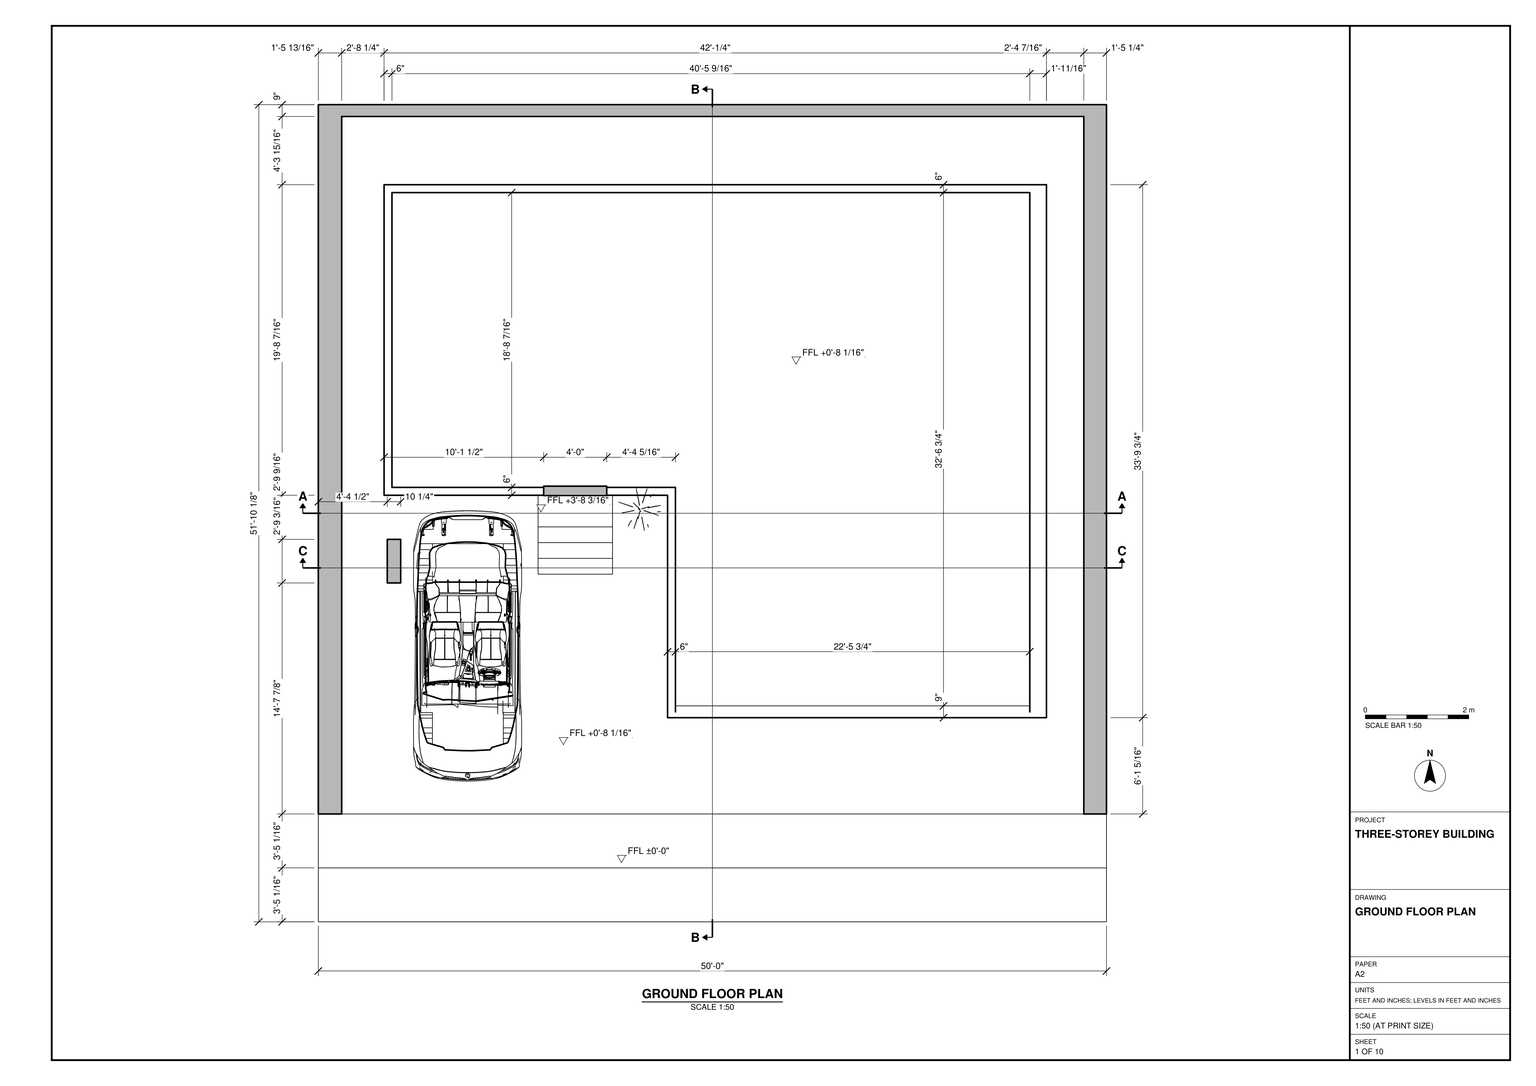
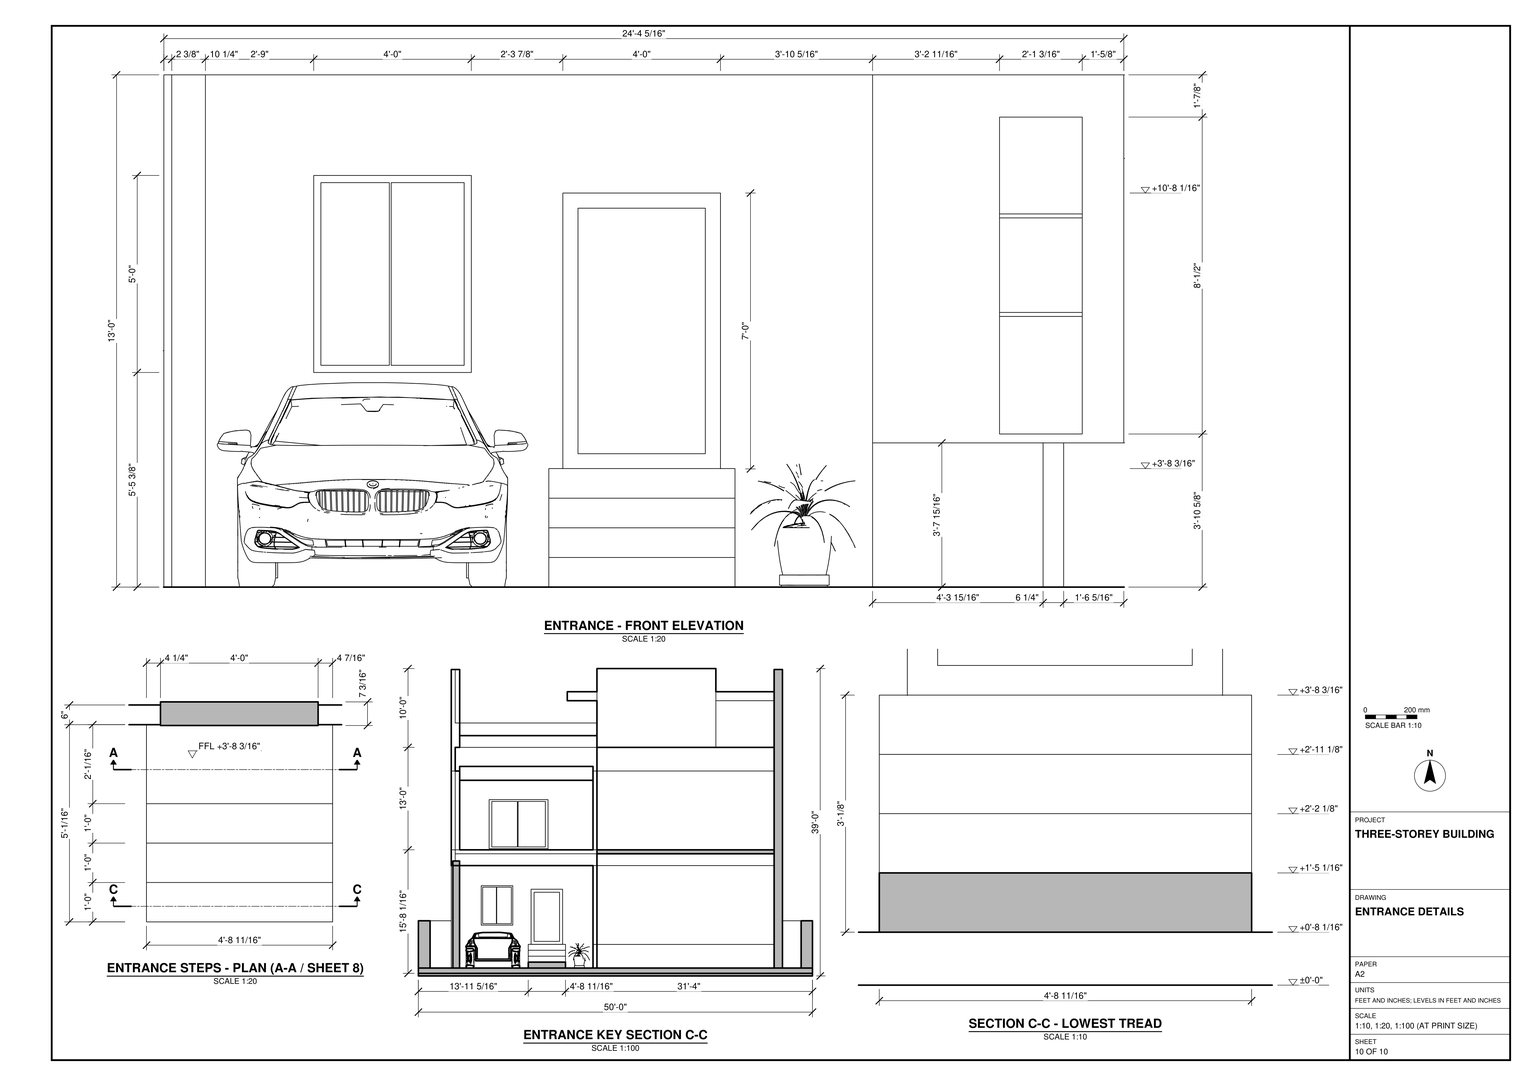
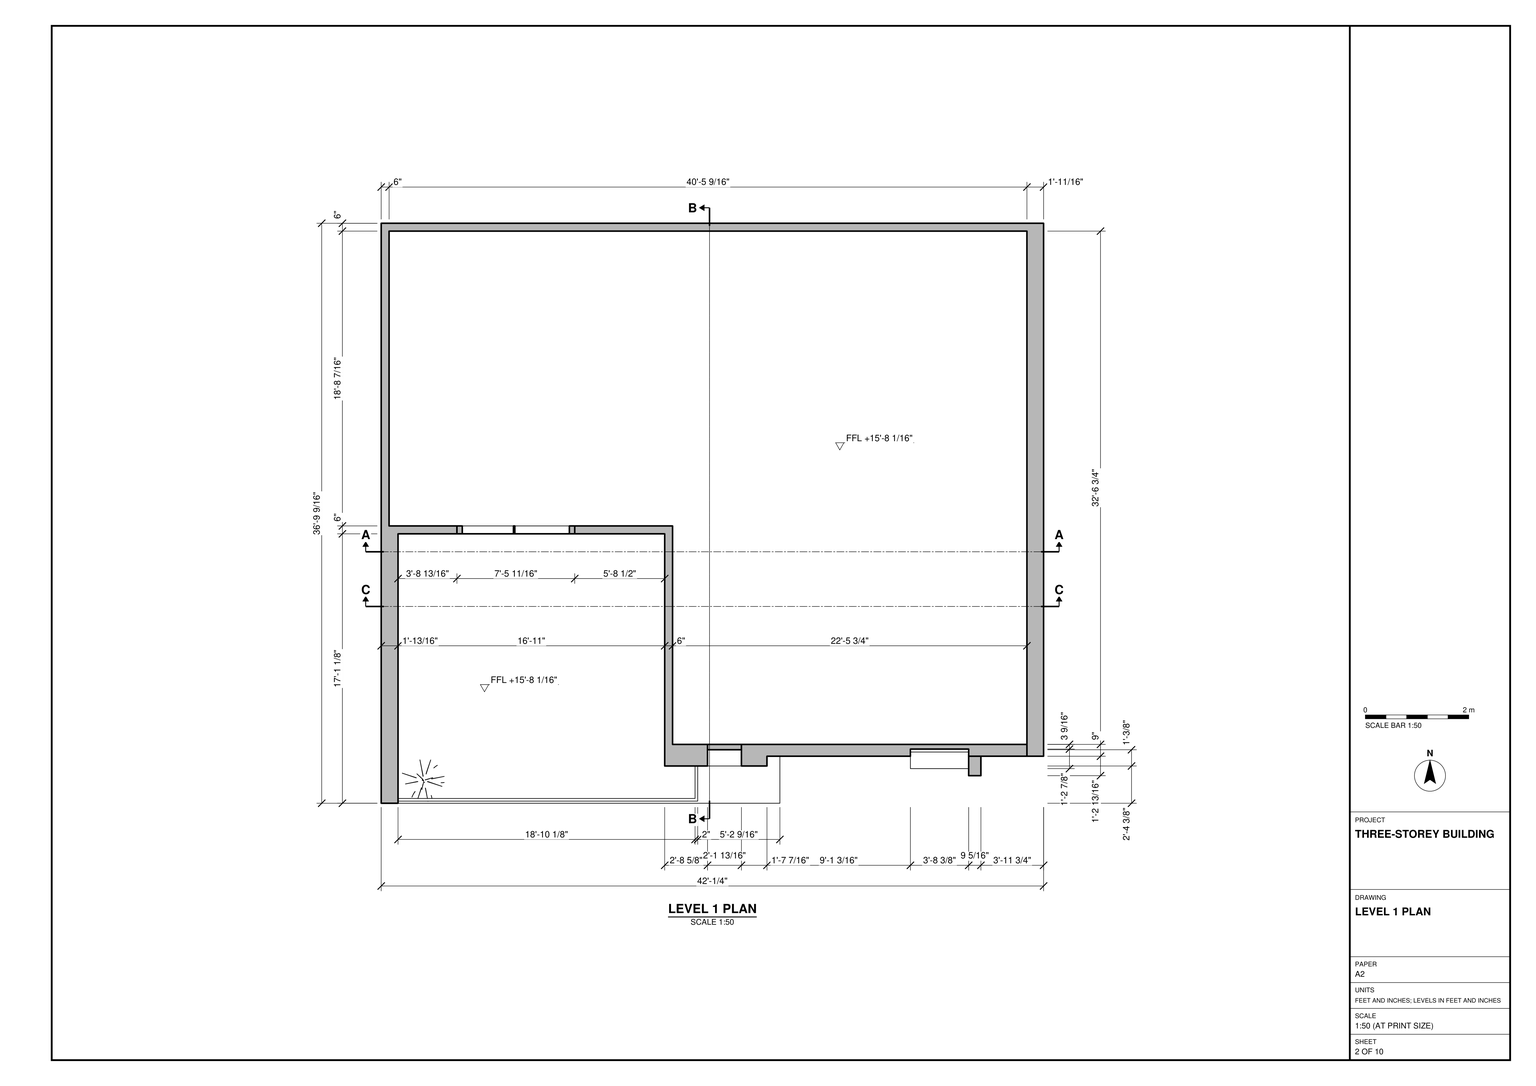
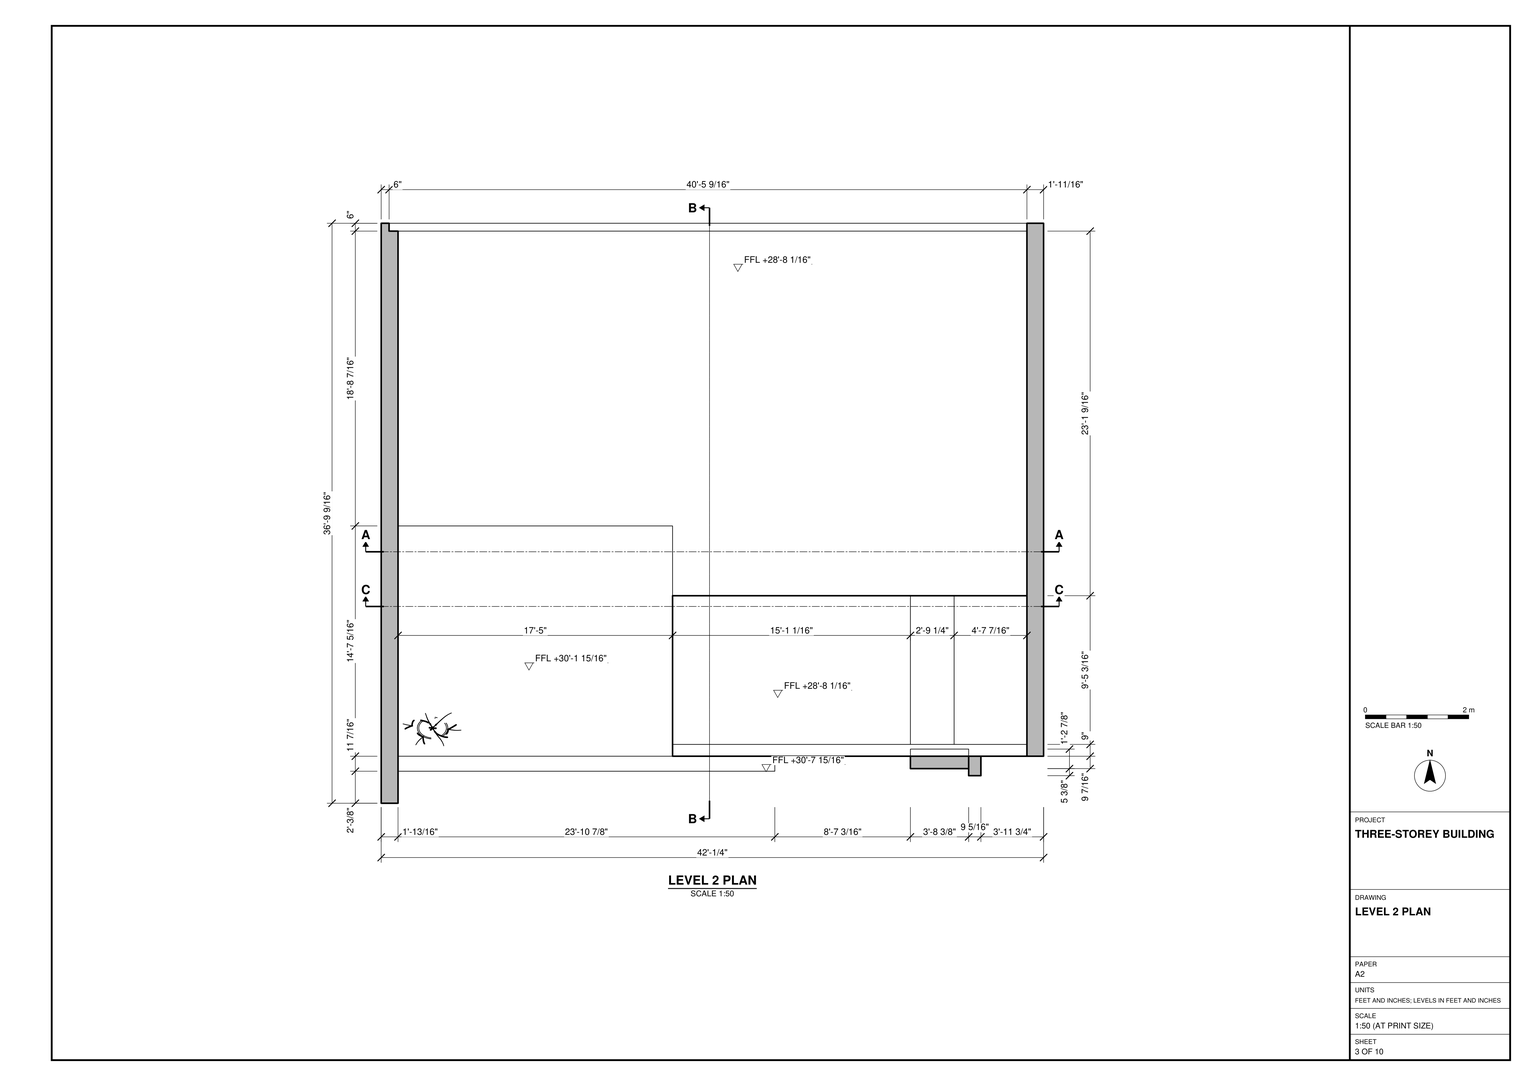
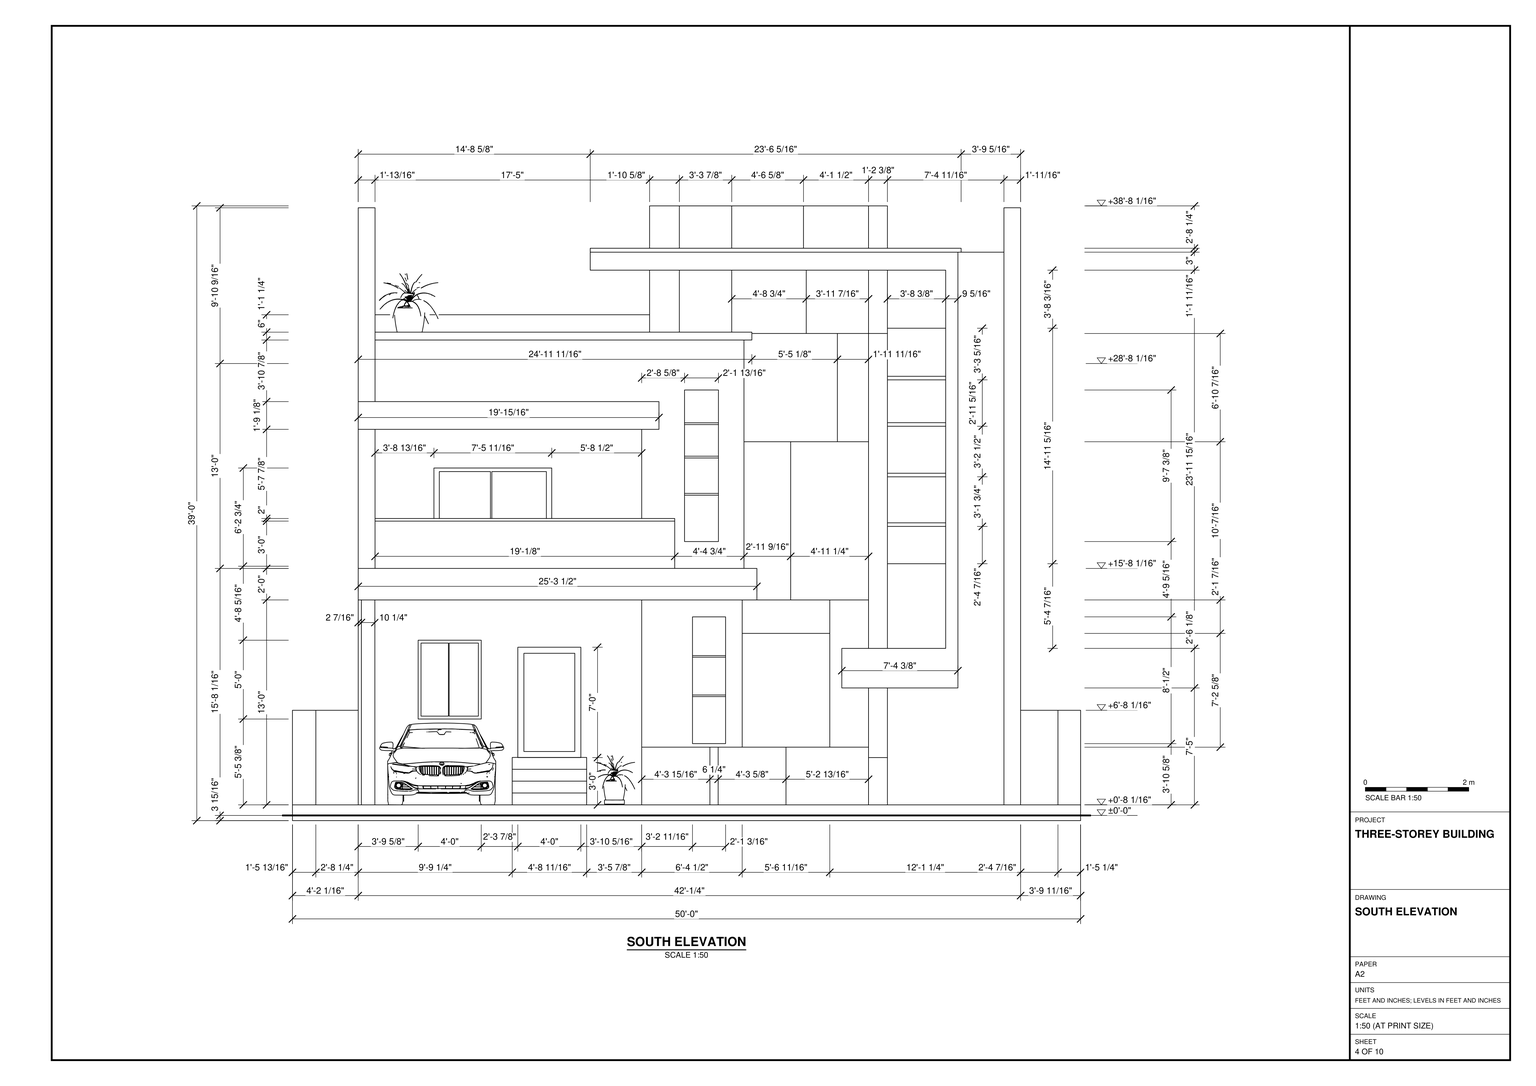
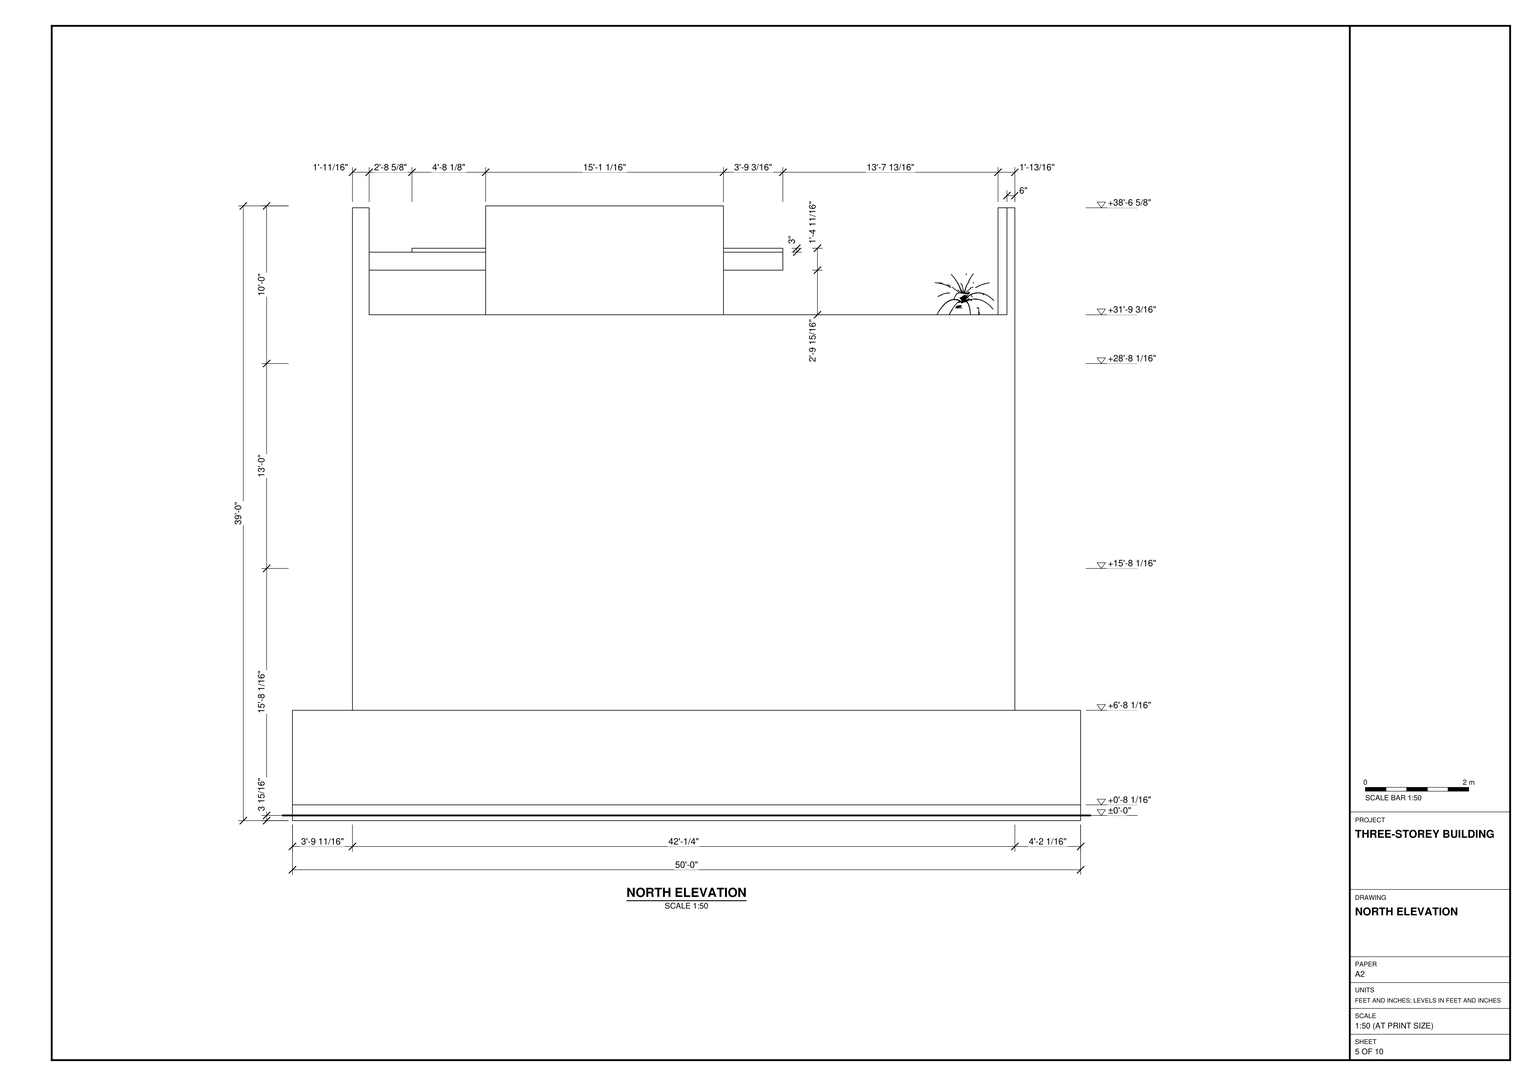
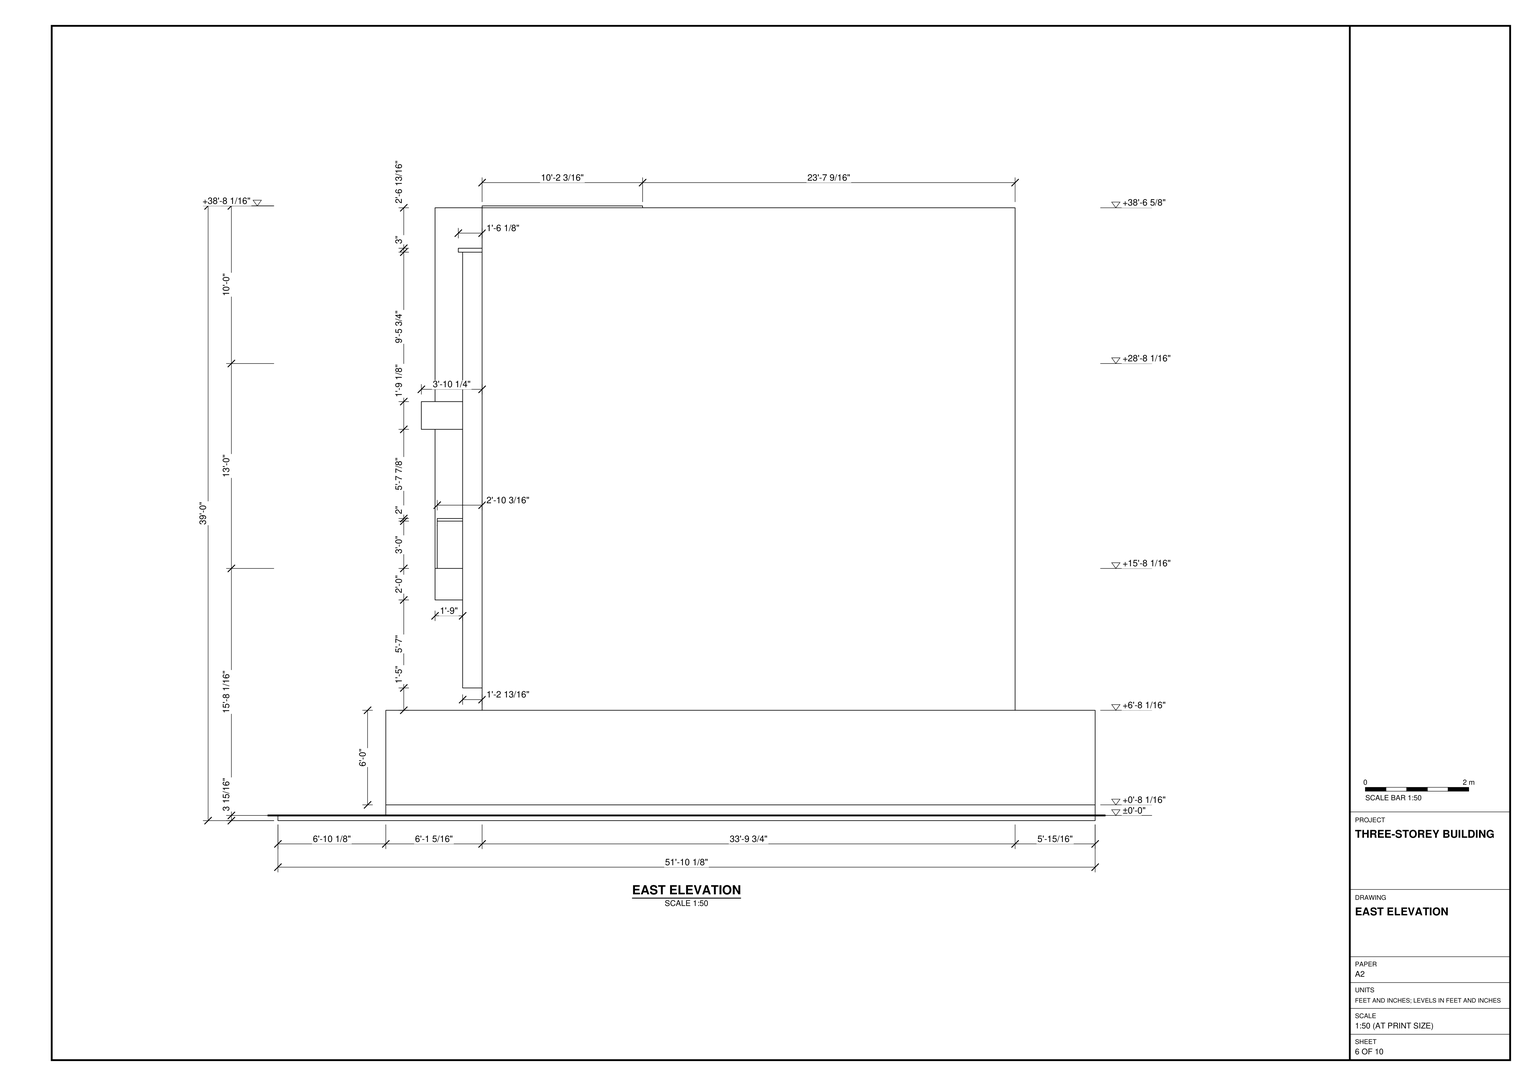
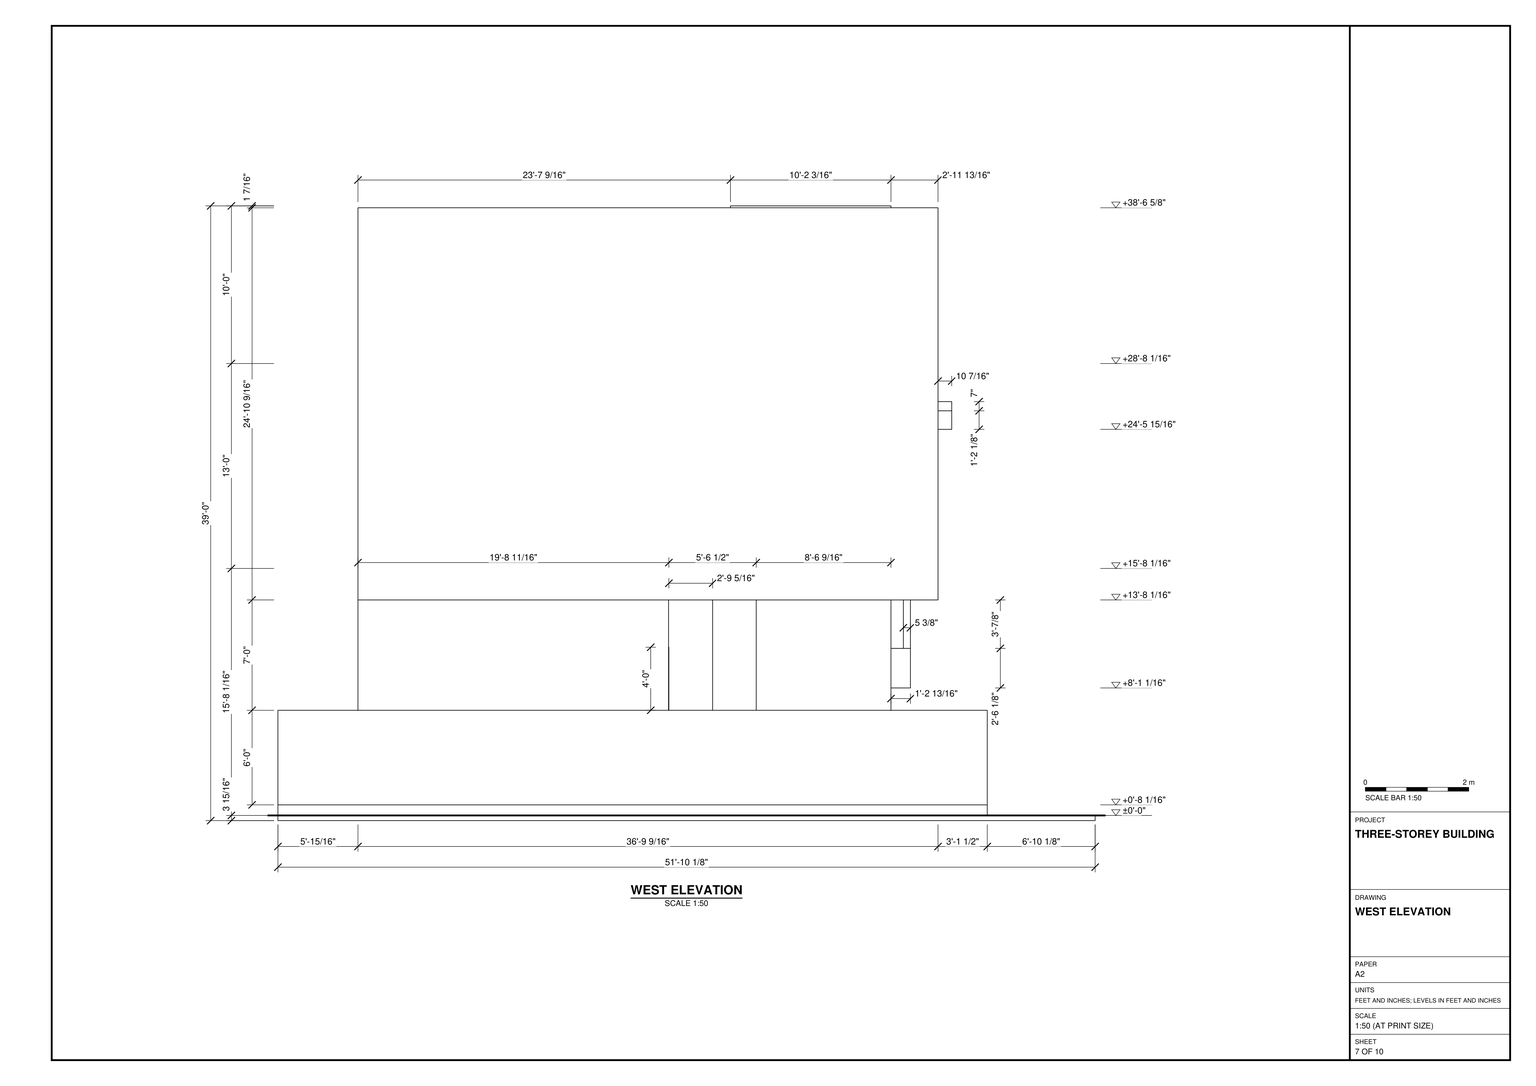
Build the three-storey building and its site in SketchUp from task_files/diagram_01.pdf. Work in feet and inches. Including the site base and front approach, the model must be 50'-0" wide, 51'-10 1/8" deep and 39'-0" high. Use ±0'-0" as the ground datum and place the upper floors at +15'-8 1/16" and +28'-8 1/16".

Trace the building footprint separately from the site boundary. The front-left recess accommodates a parked car and a flight of steps, while the right-hand wing projects towards the street. Set the parking surface at +0'-8 1/16" and bring the steps up to the entrance landing at +3'-8 3/16". Use the entrance detail to position the door at the head of the steps and the divided window behind the parking space.

Follow the wall thicknesses and offsets on each plan. Model the openings and their frames, the floor slabs, the terrace above the parking bay, and the upper walls and roof slabs at the heights shown in section. Include built-in joinery and main furniture where drawn. Decor and loose items, including the car and potted plants, may be any suitable library components. Keep shell elements and individual furniture or joinery pieces in separate groups or components, and use components for repeated parts. Save one SketchUp model as output_files/three_storey_building_with_recessed_entrance.skp.

# SketchUp Ruby script. Lengths in inches.
U = 1.inch
M = Sketchup.active_model
def pt(a) = Geom::Point3d.new(a.map { |v| v * U })
def face(e, loops, mat)
  f = e.add_face(loops[0].map { |a| pt(a) })
  loops[1..].each { |l| e.add_face(l.map { |a| pt(a) }).erase! }
  f.material = f.back_material = mat if mat
  f
end
# faces: each face lists its corners as indices into pts; further lists are holes
def faces(e, pts, list, mat = nil) = list.each { |f| face(e, (f[0].is_a?(Array) ? f : [f]).map { |l| l.map { |i| pts[i] } }, mat) }
# xy, xz, yz: faces in a plane at the given z, y or x. An outline is a flat list of corners, or four numbers for a rectangle; further outlines are holes
def ring(l) = l.size == 4 ? [[l[0], l[1]], [l[2], l[1]], [l[2], l[3]], [l[0], l[3]]] : l.each_slice(2).to_a
def flat(e, list, mat, &to3) = list.each { |f| face(e, (f[0].is_a?(Array) ? f : [f]).map { |l| ring(l).map { |u, v| to3.(u, v) } }, mat) }
def xy(e, z, list, mat = nil) = flat(e, list, mat) { |x, y| [x, y, z] }
def xz(e, y, list, mat = nil) = flat(e, list, mat) { |x, z| [x, y, z] }
def yz(e, x, list, mat = nil) = flat(e, list, mat) { |y, z| [x, y, z] }
def lines(e, pts, list) = list.each { |a, b| e.add_line(pt(pts[a]), pt(pts[b])) }
# prism: a flat outline (further loops are holes) pulled along v
def prism(e, loops, v, mat = nil)
  f = face(e, loops, mat); d = Geom::Vector3d.new(v.map { |x| x * U })
  f.pushpull(f.normal.samedirection?(d) ? d.length : -d.length)
end
def box(e, o, s, mat = nil) = prism(e, [[o, [o[0] + s[0], o[1], o[2]], [o[0] + s[0], o[1] + s[1], o[2]], [o[0], o[1] + s[1], o[2]]]], [0, 0, s[2]], mat)
def at(x, y, z, deg = 0) = Geom::Transformation.translation(pt([x, y, z])) * Geom::Transformation.rotation(ORIGIN, Z_AXIS, deg.degrees)
def axes(o, x, y, z) = Geom::Transformation.new([*x, 0, *y, 0, *z, 0, *pt(o).to_a, 1])
def part(name) = M.definitions.add(name)
# library, detail: a bought-in or finely detailed component or shape, given as its bounding box
def library(name, o, s) = part(name).tap { |d| box(d.entities, o, s) }
def detail(e, o, s) = box(e.add_group.entities, o, s)
def put(e, d, t, mat = nil) = e.add_instance(d, t).tap { |i| i.material = mat if mat }
def group(e, t, mat = nil) = e.add_group.tap { |g| g.transformation = t; g.material = mat if mat }.entities
root = M.entities
M.materials.add("[Blacktop Old 01]").color = [132, 136, 139]
M.materials.add("[Carrera Marble]").color = [207, 207, 207]
M.materials.add("[Color A08]").color = [102, 0, 0]
M.materials.add("[Color C08]").color = [102, 51, 0]
M.materials.add("[Color M00]").color = [255, 255, 255]
M.materials.add("[Color M07]").color = [58, 58, 58]
M.materials.add("[Concrete Scored Jointless]").color = [140, 133, 127]
M.materials.add("[Grass Dark Green]").color = [106, 157, 55]
M.materials.add("[Metal Seamed]").color = [118, 119, 115]
M.materials.add("[Pavers Flagstone Gray]").color = [162, 162, 162]
M.materials.add("[Stone Sandstone Ashlar Light]").color = [206, 178, 128]
M.materials.add("[Translucent Glass Gray]").color = [128, 128, 128]
M.materials["[Translucent Glass Gray]"].alpha = 0.5
M.materials.add("[Translucent Glass Safety]").color = [227, 235, 65]
M.materials["[Translucent Glass Safety]"].alpha = 0.55
M.materials.add("[Translucent Glass Safety]1").color = [255, 255, 55]
M.materials["[Translucent Glass Safety]1"].alpha = 0.5
M.materials.add("[Wood Floor Parquet]").color = [145, 89, 39]
M.materials.add("[Wood Floor]").color = [99, 57, 32]
M.materials.add("[Wood Lumber ButtJoined]").color = [190, 160, 115]
c1 = library("plants",[-16.3,-15.81,0],[32.6,31.62,37.8])
c2 = part("Group\#3")
xy(c2.entities,0,[[0,0,48,6]],"[Color A08]")
xy(c2.entities,2.1875,[[2.1875,0,23.03,6],[23.59,0,45.8125,6]],"[Color A08]")
xy(c2.entities,57.8125,[[2.1875,0,23.03,6],[23.59,0,45.8125,6]],"[Color A08]")
xy(c2.entities,60,[[0,0,48,6]],"[Color A08]")
xz(c2.entities,0,[[[0,0,48,60],[23.59,2.1875,45.8125,57.8125],[2.1875,2.1875,23.03,57.8125]]],"[Color A08]")
xz(c2.entities,0,[[2.1875,2.1875,23.03,57.8125],[23.59,2.1875,45.8125,57.8125]],"[Translucent Glass Safety]")
xz(c2.entities,6,[[[0,0,48,60],[23.59,2.1875,45.8125,57.8125],[2.1875,2.1875,23.03,57.8125]]],"[Color A08]")
yz(c2.entities,0,[[0,0,6,60]],"[Color A08]")
yz(c2.entities,2.1875,[[0,2.1875,6,57.8125]],"[Color A08]")
yz(c2.entities,23.03,[[0,2.1875,6,57.8125]],"[Color A08]")
yz(c2.entities,23.59,[[0,2.1875,6,57.8125]],"[Color A08]")
yz(c2.entities,45.8125,[[0,2.1875,6,57.8125]],"[Color A08]")
yz(c2.entities,48,[[0,0,6,60]],"[Color A08]")
c3 = library("Group\#16",[0,0,0],[94.66,205.86,62.27])
xy(root,0,[[0,0,600,622.125]])
xy(root,3.9375,[[0,82.125,600,622.125]])
xy(root,3.9375,[[0,41.0625,600,82.125]],"[Grass Dark Green]")
xy(root,3.9375,[[0,0,600,41.0625]],"[Pavers Flagstone Gray]")
xy(root,12,[[0,82.125,17.8125,82.125,17.8125,613.125,582.75,613.125,582.75,82.125,600,82.125,600,622.125,0,622.125],[[265.875,155.4375,265.875,324.75,50.0625,324.75,50.0625,561.1875,554.3125,561.1875,554.3125,155.4375],[271.875,164.4375,541.625,164.4375,541.625,555.1875,56.0625,555.1875,56.0625,330.75,271.875,330.75]],[271.875,164.4375,541.625,164.4375,541.625,555.1875,56.0625,555.1875,56.0625,330.75,271.875,330.75]])
xy(root,12,[[[17.8125,82.125,582.75,613.125],[265.875,155.4375,265.875,324.75,50.0625,324.75,50.0625,561.1875,554.3125,561.1875,554.3125,155.4375],[52.47,258.01,62.72,291.19]]],"[Blacktop Old 01]")
xy(root,12,[[52.47,258.01,62.72,291.19]],"[Wood Lumber ButtJoined]")
xy(root,48,[[171.56,324.75,219.56,330.75]])
xy(root,58.625,[[304.53,155.4375,329.72,159.8125],[304.53,159.8125,329.72,164.6875]])
xy(root,77.35,[[95.69,324.75,143.69,330.75]])
xy(root,84,[[0,82.125,17.8125,82.125,17.8125,613.125,582.75,613.125,582.75,82.125,600,82.125,600,622.125,0,622.125]])
xy(root,94.43,[[304.53,157.8125,329.72,159.8125]],"[Color C08]")
xy(root,95.64,[[304.53,157.8125,329.72,159.8125]],"[Color C08]")
xy(root,101,[[418.21,140.625,452.92,155.4375],[452.92,140.625,506.59,155.4375]],"[Color M07]")
xy(root,124.43,[[304.53,157.8125,329.72,159.8125]],"[Color C08]")
xy(root,125.64,[[304.53,157.8125,329.72,159.8125]],"[Color C08]")
xy(root,131.125,[[452.92,140.625,497.27,146],[452.92,146,497.27,155.4375]])
xy(root,131.125,[[418.21,140.625,452.92,155.4375]],"[Color M07]")
xy(root,132,[[171.56,324.75,219.56,330.75]])
xy(root,137.35,[[95.69,324.75,143.69,330.75]])
xy(root,155.125,[[304.53,155.4375,329.72,159.8125],[304.53,159.8125,306.16,164.6875],[306.16,159.8125,329.72,164.6875]])
xy(root,168,[[271.875,159.8125,541.625,164.4375]])
xy(root,168,[[50.0625,119.625,50.0625,324.75,265.875,324.75,265.875,155.4375,353.5625,155.4375,353.5625,119.625]],"[Color M07]")
xy(root,175,[[52.47,258.01,62.72,291.19]],"[Wood Lumber ButtJoined]")
xy(root,186,[[271.875,164.4375,271.875,330.75,56.0625,330.75,56.0625,555.1875,541.625,555.1875,541.625,164.4375]])
xy(root,192,[[62.875,121.25,62.875,123.25,289,123.25,289,148,291,148,291,121.25],[271.875,164.4375,541.625,164.4375,541.625,555.1875,56.0625,555.1875,56.0625,330.75,271.875,330.75]])
xy(root,192,[[62.875,119.625,353.5625,119.625,353.5625,155.4375,343.72,155.4375,343.72,148,291,148,291,121.25,62.875,121.25],[62.875,123.25,289,123.25,289,148,265.875,148,265.875,324.75,62.875,324.75]],"[Concrete Scored Jointless]")
xy(root,193.68,[[107.7,324.75,197.39,330.75]])
xy(root,195.57,[[452.92,146,497.27,160.875]])
xy(root,212.46,[[298.47,148,324.28,160.375],[298.47,160.375,324.28,164.4375]])
xy(root,223.99,[[452.92,158.625,497.27,160.875]],"[Color C08]")
xy(root,226.7,[[452.92,158.625,497.27,160.875]],"[Color C08]")
xy(root,228,[[62.875,121.25,62.875,123.25,289,123.25,289,148,291,148,291,121.25]])
xy(root,230,[[62.875,121.25,291,121.25,291,148,289,148,289,123.25,62.875,123.25]],"[Metal Seamed]")
xy(root,247.76,[[298.47,158.875,324.28,160.375]],"[Color C08]")
xy(root,249.11,[[298.47,158.875,324.28,160.375]],"[Color C08]")
xy(root,261.74,[[452.92,158.75,497.27,160.875]],"[Color C08]")
xy(root,264.45,[[452.92,158.75,497.27,160.875]],"[Color C08]")
xy(root,268.43,[[107.7,324.75,197.39,330.75]])
xy(root,276.07,[[298.47,158.875,324.28,160.375]],"[Color C08]")
xy(root,277.42,[[298.47,158.875,324.28,160.375]],"[Color C08]")
xy(root,297.875,[[50.0625,109.1875,50.0625,119.625,62.875,119.625,62.875,324.75,265.875,324.75,265.875,148,279,148,279,109.1875]],"[Wood Floor Parquet]")
xy(root,300.24,[[452.92,158.875,497.27,160.875]],"[Color C08]")
xy(root,301.51,[[298.47,158.875,324.28,160.375]],"[Color C08]")
xy(root,302.86,[[298.47,158.875,324.28,160.375]],"[Color C08]")
xy(root,302.95,[[452.92,158.875,497.27,160.875]],"[Color C08]")
xy(root,312,[[56.0625,148,62.875,324.75]])
xy(root,319,[[62.875,148,265.875,324.75]])
xy(root,319,[[50.0625,109.1875,279,109.1875,279,148,62.875,148,62.875,119.625,50.0625,119.625]],"[Wood Floor Parquet]")
xy(root,327.83,[[298.47,148,324.28,160.375],[298.47,160.375,304.53,164.4375],[304.53,160.375,324.28,164.4375]])
xy(root,335.55,[[452.92,158.875,497.27,160.875]],"[Color C08]")
xy(root,338.27,[[452.92,158.875,497.27,160.875]],"[Color C08]")
xy(root,342.625,[[56.0625,144,62.875,148]])
xy(root,348,[[56.0625,144,62.875,324.75],[271.875,164.4375,452.92,277.625],[452.92,164.4375,486.1875,277.625],[486.1875,164.4375,541.625,277.625],[271.875,277.625,541.625,277.625,541.625,555.1875,62.875,555.1875,62.875,330.75,271.875,330.75],
  [56.0625,324.75,62.875,330.75],[56.0625,330.75,62.875,555.1875]])
xy(root,365.875,[[62.875,148,343.72,155.4375],[62.875,155.4375,271.875,330.75]])
xy(root,365.875,[[62.875,144,349.72,148],[343.72,148,349.72,155.4375]],"[Wood Lumber ButtJoined]")
xy(root,371.875,[[62.875,144,349.72,155.4375]],"[Wood Lumber ButtJoined]")
xy(root,374.86,[[452.92,146,497.27,155.4375],[452.92,155.4375,497.27,160.875]])
xy(root,385.125,[[56.0625,555.1875,541.625,561.1875]])
xy(root,419.0625,[[452.92,146,497.27,155.4375]])
xy(root,419.0625,[[226.6875,140.625,343.72,155.4375],[343.72,140.625,452.92,155.4375],[452.92,140.625,497.27,146],[226.6875,155.4375,271.875,277.625]],"[Color M07]")
xy(root,432.75,[[226.6875,140.625,506.59,155.4375]])
xy(root,432.75,[[226.6875,137.3125,509.02,140.625],[506.59,140.625,509.02,155.4375],[226.6875,155.4375,271.875,277.625],[452.92,155.4375,541.625,277.625]],"[Color M07]")
xy(root,435.75,[[226.6875,137.3125,509.02,155.4375]],"[Color M07]")
xy(root,466.5625,[[50.0625,119.625,62.875,119.625,62.875,555.1875,56.0625,555.1875,56.0625,561.1875,50.0625,561.1875],[541.625,155.4375,554.3125,561.1875]])
xy(root,468,[[271.875,155.4375,452.92,277.625]],"[Carrera Marble]")
xz(root,0,[[0,0,600,3.9375]],"[Pavers Flagstone Gray]")
xz(root,82.125,[[0,12,17.8125,84],[582.75,12,600,84]],"[Color M00]")
xz(root,82.125,[[0,3.9375,600,12]],"[Grass Dark Green]")
xz(root,109.1875,[[50.0625,297.875,279,319]],"[Wood Floor Parquet]")
xz(root,119.625,[[50.0625,192,62.875,297.875],[50.0625,297.875,62.875,312],[50.0625,312,62.875,319],[50.0625,319,62.875,466.5625]])
xz(root,119.625,[[50.0625,168,353.5625,192]],"[Color M07]")
xz(root,121.25,[[62.875,228,291,230]],"[Metal Seamed]")
xz(root,121.25,[[62.875,192,291,228]],"[Translucent Glass Gray]")
xz(root,123.25,[[62.875,228,289,230]],"[Metal Seamed]")
xz(root,123.25,[[62.875,192,289,228]],"[Translucent Glass Gray]")
xz(root,137.3125,[[226.6875,432.75,509.02,435.75]],"[Color M07]")
xz(root,140.625,[[418.21,101,506.59,101,506.59,432.75,226.6875,432.75,226.6875,419.0625,497.27,419.0625,497.27,131.125,418.21,131.125]],"[Color M07]")
xz(root,144,[[56.0625,342.625,62.875,348]])
xz(root,144,[[62.875,365.875,349.72,371.875]],"[Wood Lumber ButtJoined]")
xz(root,146,[[452.92,131.125,497.27,195.57],[452.92,374.86,497.27,419.0625]])
xz(root,148,[[289,192,291,228],[289,228,291,230],[265.875,297.875,279,319],[56.0625,312,62.875,342.625]])
xz(root,148,[[[265.875,192,289,192,289,230,291,230,291,192,343.72,192,343.72,365.875,62.875,365.875,62.875,319,279,319,279,297.875,265.875,297.875],[298.47,212.46,324.28,327.83]]],"[Wood Lumber ButtJoined]")
xz(root,155.4375,[[541.625,12,554.3125,466.5625],[418.21,101,438.55,131.125],[438.55,101,438.55,131.125,497.27,131.125,497.27,419.0625,438.55,419.0625,438.55,432.75,506.59,432.75,506.59,101],[62.875,365.875,271.875,371.875],[271.875,365.875,349.72,370.87],
  [271.875,370.87,294.53,371.875],[294.53,370.87,334.4,371.875],[334.4,370.87,349.72,371.875],[452.92,374.86,497.27,419.0625],[226.6875,419.0625,294.53,432.75],
  [294.53,419.0625,334.4,432.75],[334.4,419.0625,438.55,432.75],[226.6875,432.75,271.875,435.75],[271.875,432.75,294.53,435.75],[294.53,432.75,334.4,435.75],
  [334.4,432.75,389.02,435.75],[389.02,432.75,438.55,435.75],[438.55,432.75,452.92,435.75],[452.92,432.75,509.02,435.75]])
xz(root,155.4375,[[265.875,12,317.8,55.92],[317.8,12,324.06,55.92],[324.06,12,375.71,55.92],[375.71,12,438.55,55.92],[438.55,12,452.92,48],
  [438.55,48,452.92,101],[[265.875,55.92,342.37,168],[304.53,58.625,329.72,155.125]],[342.37,55.92,409.06,142.54],[409.06,55.92,438.55,55.92,438.55,101,418.21,101,418.21,131.125,438.55,131.125,438.55,168,409.06,168],[438.55,131.125,452.92,370.87],
  [342.37,142.54,409.06,168],[353.5625,168,379.28,168,379.28,288.46,343.72,288.46,343.72,192,353.5625,192],[379.28,168,438.55,288.46],[343.72,288.46,414.84,288.46,414.84,370.87,349.72,370.87,349.72,365.875,343.72,365.875],[414.84,288.46,438.55,370.87],
  [349.72,370.87,391.13,370.87,391.13,419.0625,334.4,419.0625,334.4,371.875,349.72,371.875],[391.13,370.87,438.55,419.0625],[438.55,370.87,452.92,419.0625],[271.875,371.875,294.53,419.0625],[294.53,371.875,334.4,419.0625],
  [271.875,435.75,294.53,468],[294.53,435.75,334.4,468],[334.4,435.75,389.02,468],[389.02,435.75,438.55,468],[438.55,435.75,452.92,468]],"[Carrera Marble]")
xz(root,155.4375,[[452.92,12,541.625,12,541.625,432.75,506.59,432.75,506.59,101,452.92,101]],"[Wood Floor Parquet]")
xz(root,157.8125,[[304.53,94.43,329.72,95.64],[304.53,124.43,329.72,125.64]],"[Color C08]")
xz(root,158.625,[[452.92,223.99,497.27,226.7]],"[Color C08]")
xz(root,158.75,[[452.92,261.74,497.27,264.45]],"[Color C08]")
xz(root,158.875,[[298.47,247.76,324.28,249.11],[298.47,276.07,324.28,277.42],[452.92,300.24,497.27,302.95],[298.47,301.51,324.28,302.86],[452.92,335.55,497.27,338.27]],"[Color C08]")
xz(root,159.8125,[[304.53,58.625,329.72,94.43],[304.53,95.64,329.72,124.43],[304.53,125.64,329.72,155.125]],"[Translucent Glass Safety]1")
xz(root,160.375,[[298.47,212.46,324.28,247.76],[298.47,249.11,324.28,276.07],[298.47,277.42,324.28,301.51],[298.47,302.86,324.28,327.83]],"[Translucent Glass Safety]1")
xz(root,160.875,[[452.92,223.99,497.27,226.7],[452.92,261.74,497.27,264.45],[452.92,300.24,497.27,302.95],[452.92,335.55,497.27,338.27]],"[Color C08]")
xz(root,160.875,[[452.92,195.57,497.27,223.99],[452.92,226.7,497.27,261.74],[452.92,264.45,497.27,300.24],[452.92,302.95,497.27,335.55],[452.92,338.27,497.27,374.86]],"[Translucent Glass Safety]1")
xz(root,164.4375,[[271.875,168,541.625,186],[271.875,186,507.1875,192],[507.1875,186,541.625,192],[[271.875,192,541.625,348],[298.47,212.46,324.28,327.83]],[298.47,212.46,324.28,327.83]])
xz(root,164.6875,[[304.53,58.625,329.72,155.125]])
xz(root,199.5,[[304.53,135.16,329.72,136.37]])
xz(root,258.01,[[52.47,12,62.72,175]],"[Wood Lumber ButtJoined]")
xz(root,277.625,[[452.92,348,541.625,419.0625]])
xz(root,277.625,[[271.875,348,452.92,468]],"[Carrera Marble]")
xz(root,277.625,[[226.6875,419.0625,271.875,432.75],[452.92,419.0625,541.625,432.75]],"[Color M07]")
xz(root,291.19,[[52.47,12,62.72,175]],"[Wood Lumber ButtJoined]")
xz(root,324.75,[[62.875,297.875,265.875,319]])
xz(root,324.75,[[[50.0625,12,265.875,168],[171.56,48,219.56,132],[95.69,77.35,143.69,137.35]],[[62.875,192,265.875,297.875],[107.7,193.68,197.39,268.43]]],"[Wood Lumber ButtJoined]")
xz(root,330.75,[[56.0625,12,271.875,48],[[56.0625,48,56.0625,168,271.875,168,271.875,48,219.56,48,219.56,132,171.56,132,171.56,48],[95.69,77.35,143.69,137.35]],[56.0625,168,271.875,186],[56.0625,186,271.875,192],[[56.0625,192,271.875,312],[107.7,193.68,197.39,268.43]],
  [56.0625,312,271.875,348],[62.875,348,271.875,365.875]])
xz(root,555.1875,[[56.0625,12,541.625,48],[56.0625,48,541.625,168],[56.0625,168,541.625,186],[56.0625,186,541.625,192],[56.0625,192,541.625,312],
  [56.0625,312,541.625,348],[62.875,348,541.625,385.125],[56.0625,385.125,62.875,466.5625]])
xz(root,561.1875,[[50.0625,12,554.3125,48]])
xz(root,561.1875,[[50.0625,48,50.0625,466.5625,56.0625,466.5625,56.0625,385.125,541.625,385.125,541.625,466.5625,554.3125,466.5625,554.3125,48]],"[Stone Sandstone Ashlar Light]")
xz(root,613.125,[[17.8125,12,582.75,84]])
xz(root,622.125,[[0,0,600,3.9375],[0,3.9375,600,12],[0,12,600,84]])
yz(root,0,[[0,0,622.125,3.9375],[82.125,3.9375,622.125,12],[82.125,12,622.125,84]])
yz(root,17.8125,[[82.125,12,613.125,84]])
yz(root,50.0625,[[324.75,12,561.1875,48],[109.1875,297.875,119.625,312],[109.1875,312,119.625,319]])
yz(root,50.0625,[[324.75,48,561.1875,168],[119.625,168,561.1875,466.5625]],"[Stone Sandstone Ashlar Light]")
yz(root,52.47,[[258.01,12,291.19,175]],"[Wood Lumber ButtJoined]")
yz(root,56.0625,[[330.75,12,555.1875,48],[330.75,48,555.1875,168],[330.75,168,555.1875,186],[330.75,186,555.1875,192],[330.75,192,555.1875,312],
  [148,312,324.75,312,324.75,348,144,348,144,342.625,148,342.625],[324.75,312,330.75,348],[330.75,312,555.1875,348],[555.1875,385.125,561.1875,466.5625]])
yz(root,62.72,[[258.01,12,291.19,175]],"[Wood Lumber ButtJoined]")
yz(root,62.875,[[119.625,192,121.25,192,121.25,230,123.25,230,123.25,192,324.75,192,324.75,297.875,119.625,297.875],[121.25,192,123.25,228],[121.25,228,123.25,230],[119.625,297.875,148,312],[148,297.875,324.75,312],
  [119.625,312,148,319],[148,312,324.75,319],[119.625,319,148,319,148,342.625,144,342.625,144,371.875,155.4375,371.875,155.4375,365.875,330.75,365.875,330.75,348,555.1875,348,555.1875,466.5625,119.625,466.5625],[144,342.625,148,348],[144,348,148,365.875],
  [148,348,324.75,365.875],[324.75,348,330.75,365.875],[144,365.875,155.4375,371.875]])
yz(root,95.69,[[324.75,77.35,330.75,137.35]])
yz(root,107.7,[[324.75,193.68,330.75,268.43]])
yz(root,143.69,[[324.75,77.35,330.75,137.35]])
yz(root,171.56,[[324.75,48,330.75,132]])
yz(root,197.39,[[324.75,193.68,330.75,268.43]])
yz(root,219.56,[[324.75,48,330.75,132]])
yz(root,226.6875,[[140.625,419.0625,155.4375,432.75],[155.4375,419.0625,277.625,432.75],[137.3125,432.75,155.4375,435.75]],"[Color M07]")
yz(root,265.875,[[148,297.875,324.75,319]])
yz(root,265.875,[[155.4375,12,324.75,168],[148,192,324.75,297.875]],"[Wood Lumber ButtJoined]")
yz(root,271.875,[[164.4375,12,330.75,48],[159.8125,48,330.75,168],[164.4375,168,330.75,186],[164.4375,186,330.75,192],[164.4375,192,330.75,312],
  [164.4375,312,330.75,348],[164.4375,348,277.625,365.875],[277.625,348,330.75,365.875]])
yz(root,271.875,[[155.4375,365.875,277.625,419.0625],[155.4375,432.75,277.625,468]],"[Carrera Marble]")
yz(root,279,[[109.1875,297.875,148,319]],"[Wood Floor Parquet]")
yz(root,289,[[123.25,228,148,230]],"[Metal Seamed]")
yz(root,289,[[123.25,192,148,228]],"[Translucent Glass Gray]")
yz(root,291,[[121.25,228,148,230]],"[Metal Seamed]")
yz(root,291,[[121.25,192,148,228]],"[Translucent Glass Gray]")
yz(root,298.47,[[148,212.46,160.375,212.46,160.375,247.76,158.875,247.76,158.875,249.11,160.375,249.11,160.375,276.07,158.875,276.07,158.875,277.42,160.375,277.42,160.375,301.51,158.875,301.51,158.875,302.86,160.375,302.86,160.375,327.83,148,327.83],[160.375,212.46,164.4375,212.46,164.4375,327.83,160.375,327.83,160.375,302.86,158.875,302.86,158.875,301.51,160.375,301.51,160.375,277.42,158.875,277.42,158.875,276.07,160.375,276.07,160.375,249.11,158.875,249.11,158.875,247.76,160.375,247.76]])
yz(root,304.53,[[155.4375,58.625,159.8125,58.625,159.8125,94.43,157.8125,94.43,157.8125,95.64,159.8125,95.64,159.8125,124.43,157.8125,124.43,157.8125,125.64,159.8125,125.64,159.8125,155.125,155.4375,155.125],[159.8125,58.625,159.8125,94.43,157.8125,94.43,157.8125,95.64,159.8125,95.64,159.8125,124.43,157.8125,124.43,157.8125,125.64,159.8125,125.64,159.8125,155.125,164.6875,155.125,164.6875,58.625]])
yz(root,324.28,[[148,212.46,148,327.83,160.375,327.83,160.375,302.86,158.875,302.86,158.875,301.51,160.375,301.51,160.375,277.42,158.875,277.42,158.875,276.07,160.375,276.07,160.375,249.11,158.875,249.11,158.875,247.76,160.375,247.76,160.375,212.46],[160.375,212.46,160.375,247.76,158.875,247.76,158.875,249.11,160.375,249.11,160.375,276.07,158.875,276.07,158.875,277.42,160.375,277.42,160.375,301.51,158.875,301.51,158.875,302.86,160.375,302.86,160.375,327.83,164.4375,327.83,164.4375,212.46]])
yz(root,329.72,[[155.4375,58.625,155.4375,155.125,159.8125,155.125,159.8125,125.64,157.8125,125.64,157.8125,124.43,159.8125,124.43,159.8125,95.64,157.8125,95.64,157.8125,94.43,159.8125,94.43,159.8125,58.625],[159.8125,58.625,164.6875,58.625,164.6875,155.125,159.8125,155.125,159.8125,125.64,157.8125,125.64,157.8125,124.43,159.8125,124.43,159.8125,95.64,157.8125,95.64,157.8125,94.43,159.8125,94.43]])
yz(root,343.72,[[148,192,155.4375,365.875]],"[Wood Lumber ButtJoined]")
yz(root,349.72,[[144,365.875,155.4375,371.875]],"[Wood Lumber ButtJoined]")
yz(root,353.5625,[[119.625,168,155.4375,192]],"[Color M07]")
yz(root,418.21,[[140.625,101,155.4375,131.125]],"[Color M07]")
yz(root,452.92,[[146,131.125,155.4375,195.57],[146,374.86,155.4375,419.0625]])
yz(root,452.92,[[155.4375,432.75,277.625,468]],"[Carrera Marble]")
yz(root,452.92,[[158.625,223.99,160.875,226.7],[158.75,261.74,160.875,264.45],[158.875,300.24,160.875,302.95],[158.875,335.55,160.875,338.27]],"[Color C08]")
yz(root,452.92,[[155.4375,195.57,160.875,195.57,160.875,223.99,158.625,223.99,158.625,226.7,160.875,226.7,160.875,261.74,158.75,261.74,158.75,264.45,160.875,264.45,160.875,300.24,158.875,300.24,158.875,302.95,160.875,302.95,160.875,335.55,158.875,335.55,158.875,338.27,160.875,338.27,160.875,374.86,155.4375,374.86]],"[Color M07]")
yz(root,497.27,[[146,131.125,155.4375,195.57],[146,374.86,155.4375,419.0625]])
yz(root,497.27,[[158.625,223.99,160.875,226.7],[158.75,261.74,160.875,264.45],[158.875,300.24,160.875,302.95],[158.875,335.55,160.875,338.27]],"[Color C08]")
yz(root,497.27,[[140.625,131.125,140.625,312,155.4375,312,155.4375,195.57,146,195.57,146,131.125],[155.4375,195.57,155.4375,312,160.875,312,160.875,302.95,158.875,302.95,158.875,300.24,160.875,300.24,160.875,264.45,158.75,264.45,158.75,261.74,160.875,261.74,160.875,226.7,158.625,226.7,158.625,223.99,160.875,223.99,160.875,195.57],[140.625,312,155.4375,348],[155.4375,312,155.4375,348,160.875,348,160.875,338.27,158.875,338.27,158.875,335.55,160.875,335.55,160.875,312],[140.625,348,140.625,419.0625,146,419.0625,146,374.86,155.4375,374.86,155.4375,348],
  [155.4375,348,160.875,374.86]],"[Color M07]")
yz(root,506.59,[[140.625,101,155.4375,432.75]],"[Color M07]")
yz(root,509.02,[[137.3125,432.75,155.4375,435.75]],"[Color M07]")
yz(root,541.625,[[164.4375,12,555.1875,48],[159.8125,48,555.1875,168],[155.4375,168,164.4375,192],[164.4375,168,555.1875,186],[164.4375,186,555.1875,192],
  [155.4375,192,164.4375,312],[164.4375,192,555.1875,312],[155.4375,312,164.4375,348],[164.4375,312,555.1875,348],[155.4375,348,277.625,419.0625],
  [277.625,348,277.625,432.75,164.4375,432.75,164.4375,466.5625,555.1875,466.5625,555.1875,348],[555.1875,385.125,561.1875,466.5625],[155.4375,419.0625,277.625,432.75],[155.4375,432.75,164.4375,466.5625]])
yz(root,554.3125,[[155.4375,12,561.1875,466.5625]],"[Stone Sandstone Ashlar Light]")
yz(root,582.75,[[82.125,12,613.125,84]])
yz(root,600,[[0,0,622.125,3.9375],[82.125,3.9375,622.125,12],[82.125,12,622.125,84]])
p = [[50.0625,324.75,312],[56.0625,324.75,312],[50.0625,324.75,192],[62.875,324.75,192]]
lines(root,p,[[0,1],[2,3]])
put(root,c1,at(244.88,313.88,12))
put(root,c1,at(82.36,136.9,192))
put(root,c1,axes([88.875,176.75,365.875],[1.4,0,0],[0,1,0],[0,0,1.35]))
g1 = group(root,at(167.29,264.6875,12))
prism(g1,[[[56.6875,36,36.1],[56.6875,36,27.07],[56.6875,24,27.07],[56.6875,24,18.05],[56.6875,12,18.05],[56.6875,12,9.02],[56.6875,0,9.02],[56.6875,0,0],[56.6875,12,0],[56.6875,60.0625,0],[56.6875,60.0625,36.1]]],[-56.6875,0,0])
put(root,c2,at(95.69,324.75,77.35))
put(root,c2,axes([107.7,324.75,193.68],[1.86849,0,0],[0,1,0],[0,0,1.24583]))
g2 = group(root,at(171.56,324.5,48))
xy(g2,0,[[0,0,48,7.1875]],"[Wood Floor]")
xy(g2,4.61,[[4.61,3.5,43.39,7.1875]])
xy(g2,4.61,[[4.61,0,43.39,3.5]],"[Wood Floor]")
xy(g2,79.39,[[4.61,3.5,43.39,7.1875]])
xy(g2,79.39,[[4.61,0,43.39,3.5]],"[Wood Floor]")
xy(g2,84,[[0,0,48,7.1875]],"[Wood Floor]")
xz(g2,0,[[[0,0,48,84],[4.61,4.61,43.39,79.39]]],"[Wood Floor]")
xz(g2,3.5,[[4.61,4.61,43.39,79.39]],"[Wood Floor]")
xz(g2,7.1875,[[[0,0,48,84],[4.61,4.61,43.39,79.39]],[4.61,4.61,43.39,79.39]],"[Wood Floor]")
yz(g2,0,[[0,0,7.1875,84]],"[Wood Floor]")
yz(g2,4.61,[[3.5,4.61,7.1875,79.39]])
yz(g2,4.61,[[0,4.61,3.5,79.39]],"[Wood Floor]")
yz(g2,43.39,[[3.5,4.61,7.1875,79.39]])
yz(g2,43.39,[[0,4.61,3.5,79.39]],"[Wood Floor]")
yz(g2,48,[[0,0,7.1875,84]],"[Wood Floor]")
put(root,c3,at(66.29,107.14,12))
